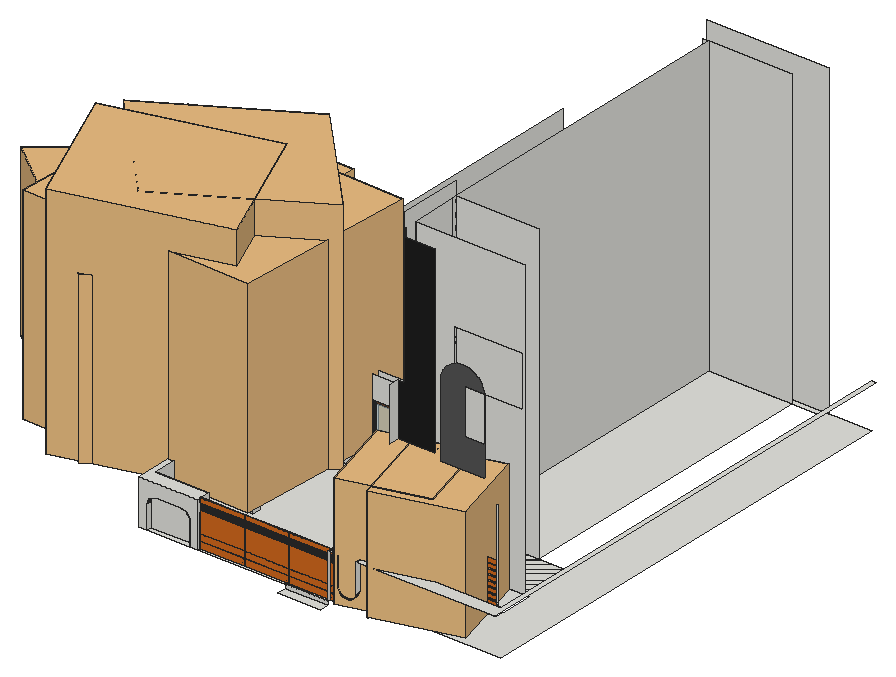
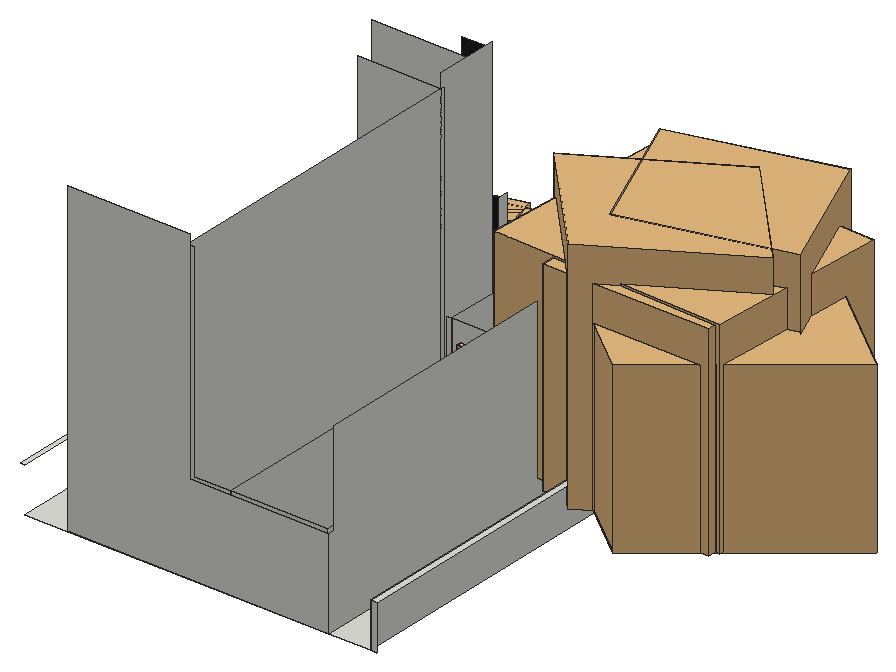
# SketchUp Ruby script. Lengths in inches.
U = 1.inch
M = Sketchup.active_model
def pt(a) = Geom::Point3d.new(a.map { |v| v * U })
def face(e, loops, mat)
  f = e.add_face(loops[0].map { |a| pt(a) })
  loops[1..].each { |l| e.add_face(l.map { |a| pt(a) }).erase! }
  f.material = f.back_material = mat if mat
  f
end
# faces: each face lists its corners as indices into pts; further lists are holes
def faces(e, pts, list, mat = nil) = list.each { |f| face(e, (f[0].is_a?(Array) ? f : [f]).map { |l| l.map { |i| pts[i] } }, mat) }
# xy, xz, yz: faces in a plane at the given z, y or x. An outline is a flat list of corners, or four numbers for a rectangle; further outlines are holes
def ring(l) = l.size == 4 ? [[l[0], l[1]], [l[2], l[1]], [l[2], l[3]], [l[0], l[3]]] : l.each_slice(2).to_a
def flat(e, list, mat, &to3) = list.each { |f| face(e, (f[0].is_a?(Array) ? f : [f]).map { |l| ring(l).map { |u, v| to3.(u, v) } }, mat) }
def xy(e, z, list, mat = nil) = flat(e, list, mat) { |x, y| [x, y, z] }
def xz(e, y, list, mat = nil) = flat(e, list, mat) { |x, z| [x, y, z] }
def yz(e, x, list, mat = nil) = flat(e, list, mat) { |y, z| [x, y, z] }
def lines(e, pts, list) = list.each { |a, b| e.add_line(pt(pts[a]), pt(pts[b])) }
# prism: a flat outline (further loops are holes) pulled along v
def prism(e, loops, v, mat = nil)
  f = face(e, loops, mat); d = Geom::Vector3d.new(v.map { |x| x * U })
  f.pushpull(f.normal.samedirection?(d) ? d.length : -d.length)
end
def box(e, o, s, mat = nil) = prism(e, [[o, [o[0] + s[0], o[1], o[2]], [o[0] + s[0], o[1] + s[1], o[2]], [o[0], o[1] + s[1], o[2]]]], [0, 0, s[2]], mat)
def at(x, y, z, deg = 0) = Geom::Transformation.translation(pt([x, y, z])) * Geom::Transformation.rotation(ORIGIN, Z_AXIS, deg.degrees)
def axes(o, x, y, z) = Geom::Transformation.new([*x, 0, *y, 0, *z, 0, *pt(o).to_a, 1])
def part(name) = M.definitions.add(name)
# library, detail: a bought-in or finely detailed component or shape, given as its bounding box
def library(name, o, s) = part(name).tap { |d| box(d.entities, o, s) }
def detail(e, o, s) = box(e.add_group.entities, o, s)
def put(e, d, t, mat = nil) = e.add_instance(d, t).tap { |i| i.material = mat if mat }
def group(e, t, mat = nil) = e.add_group.tap { |g| g.transformation = t; g.material = mat if mat }.entities
root = M.entities
M.materials.add("[0041_Chocolate]").color = [210, 105, 30]
M.materials.add("[Color M06]").color = [84, 84, 84]
M.materials.add("[Color M08]").color = [30, 30, 30]
M.materials.add("[Translucent Glass Safety]").color = [204, 235, 244]
M.materials["[Translucent Glass Safety]"].alpha = 0.5
M.materials.add("[Wood Veneer 01]").color = [120, 70, 37]
M.materials.add("[Wood Veneer 01]2").color = [94, 55, 29]
c1 = library("Group\#287",[-33.32,-34.9375,32.67],[162.87,159.66,128.34])
c2 = library("Group\#288",[-10.45,-6.67,0],[121.7,116.61,164.95])
c3 = library("Group\#286",[-10.45,-6.67,0],[121.7,116.61,164.95])
c4 = library("Group\#284",[-10.45,-6.67,0],[121.7,116.61,164.95])
c5 = library("Group\#283",[-33.32,-34.9375,32.67],[162.87,159.66,128.34])
c6 = library("Group\#285",[-33.32,-34.9375,81.35],[162.87,159.66,79.66])
c7 = library("Group\#282",[-33.32,-34.9375,77.91],[162.87,159.66,83.1])
c8 = part("Palem Elek")
put(c8.entities,c1,axes([92.2,20.3,-29.73],[0.70711,0.70711,0],[-0.70711,0.70711,0],[0,0,0.91208]))
put(c8.entities,c2,axes([60.27,20.78,0],[1,0,0],[0,1,0],[0,0,0.85762]))
put(c8.entities,c3,at(25.45,60.83,0,-53.5))
put(c8.entities,c4,at(84.4375,135.48,0,-161.4))
put(c8.entities,c5,axes([38.54,105.7,-36.19],[-0.04013,-0.99919,0],[0.99919,-0.04013,0],[0,0,1.11001]))
put(c8.entities,c6,axes([57.15,96.51,-54.45],[-0.02003,-0.49872,0.02965],[0.4996,-0.02007,0],[0.00123,0.03065,0.51628]))
put(c8.entities,c7,axes([74.94,50.39,-54.06],[0.40095,0.29715,0.03075],[-0.29654,0.38966,0.10114],[0.04012,-0.11026,0.54246]))
c9 = part("palem elek\#1")
put(c9.entities,c8,at(-81.14,-74.56,-0.83))
c10 = part("Coqueiro")
put(c10.entities,c9,axes([83.17,89.39,9.5625],[0,1.1016,0],[-1.377,0,0],[0,0,1.39284]))
c11 = part("Slatted screen panel")
xy(c11.entities,0,[[0,0,255.91,1.97]],"[Wood Veneer 01]2")
xy(c11.entities,16.54,[[0,1.18,255.91,1.97]],"[Wood Veneer 01]2")
xy(c11.entities,16.93,[[0,0,255.91,1.18]],"[Wood Veneer 01]2")
xy(c11.entities,17.78,[[0,0,255.91,1.18]],"[Wood Veneer 01]2")
xy(c11.entities,34.45,[[0,0,255.91,1.18]],"[Wood Veneer 01]2")
xy(c11.entities,35.07,[[0,0,255.91,1.18]],"[Wood Veneer 01]2")
xy(c11.entities,89.37,[[0,0,255.91,1.97]],"[Wood Veneer 01]2")
xy(c11.entities,92.91,[[0,0,255.91,1.97]],"[Wood Veneer 01]2")
xy(c11.entities,94.49,[[0,0,255.91,1.97]],"[Wood Veneer 01]2")
xy(c11.entities,97.64,[[0,0,255.91,1.97]],"[Wood Veneer 01]2")
xy(c11.entities,99.21,[[0,0,255.91,1.97]],"[Wood Veneer 01]2")
xy(c11.entities,102.36,[[0,0,255.91,1.97]],"[Wood Veneer 01]2")
xy(c11.entities,103.9375,[[0,0,255.91,1.97]],"[Wood Veneer 01]2")
xy(c11.entities,107.48,[[0,0,255.91,1.97]],"[Wood Veneer 01]2")
xy(c11.entities,119.29,[[0,0,255.91,1.97]],"[Wood Veneer 01]2")
xz(c11.entities,0,[[0,0,255.91,16.93],[0,17.78,255.91,34.45],[0,35.07,255.91,89.37],[0,92.91,255.91,94.49],[0,97.64,255.91,99.21],
  [0,102.36,255.91,103.9375],[0,107.48,255.91,119.29]],"[0041_Chocolate]")
xz(c11.entities,1.18,[[0,16.54,255.91,16.93],[0,16.93,255.91,17.78],[0,34.45,255.91,35.07]],"[Wood Veneer 01]2")
xz(c11.entities,1.97,[[0,0,255.91,1.57],[0,1.57,255.91,5.51],[0,5.51,255.91,7.09],[0,7.09,255.91,11.8125],[0,11.8125,255.91,16.54],
  [0,16.54,255.91,19.69],[0,19.69,255.91,89.37],[0,92.91,255.91,94.49],[0,97.64,255.91,99.21],[0,102.36,255.91,103.9375],
  [0,107.48,255.91,109.84],[0,109.84,255.91,119.29]],"[Wood Veneer 01]2")
yz(c11.entities,0,[[0,0,1.97,1.57],[0,1.57,1.97,5.51],[0,5.51,1.97,7.09],[0,7.09,1.97,11.8125],[0,11.8125,0,16.93,1.18,16.93,1.18,16.54,1.97,16.54,1.97,11.8125],
  [1.18,16.54,1.97,19.69],[0,17.78,0,34.45,1.18,34.45,1.18,35.07,0,35.07,0,89.37,1.97,89.37,1.97,19.69,1.18,19.69,1.18,17.78],[0,92.91,1.97,94.49],[0,97.64,1.97,99.21],[0,102.36,1.97,103.9375],
  [0,107.48,1.97,109.84],[0,109.84,1.97,119.29]],"[Wood Veneer 01]2")
yz(c11.entities,255.91,[[0,0,1.97,1.57],[0,1.57,1.97,5.51],[0,5.51,1.97,7.09],[0,7.09,1.97,11.8125],[0,11.8125,1.97,11.8125,1.97,16.54,1.18,16.54,1.18,16.93,0,16.93],
  [1.18,16.54,1.97,19.69],[0,17.78,1.18,17.78,1.18,19.69,1.97,19.69,1.97,89.37,0,89.37,0,35.07,1.18,35.07,1.18,34.45,0,34.45],[0,92.91,1.97,94.49],[0,97.64,1.97,99.21],[0,102.36,1.97,103.9375],
  [0,107.48,1.97,109.84],[0,109.84,1.97,119.29]],"[Wood Veneer 01]2")
p = [[255.91,1.97,103.9375],[255.91,1.97,107.48],[0,1.97,107.48],[0,1.97,103.9375],[0,1.97,92.91],[0,1.97,89.37],
  [255.91,1.97,99.21],[255.91,1.97,102.36],[255.91,1.97,89.37],[255.91,1.97,92.91],[0,1.97,97.64],[0,1.97,94.49],
  [0,1.97,102.36],[0,1.97,99.21],[255.91,1.97,94.49],[255.91,1.97,97.64],[240.94,0,5.51],[240.94,1.97,5.51]]
lines(c11.entities,p,[[0,1],[2,3],[4,5],[6,7],[8,9],[10,11],[12,13],[14,15],[16,17]])
c12 = part("Group\#3")
g1 = group(c12.entities,at(0,0,0))
xy(g1,0,[[0,0,6,48]],"[Wood Veneer 01]")
xy(g1,4,[[0,4,1.8125,44],[1.8125,4,6,44]])
xy(g1,80,[[0,4,1.8125,44],[1.8125,4,6,44]])
xy(g1,84,[[0,0,6,48]],"[Wood Veneer 01]")
xz(g1,0,[[0,0,6,84]],"[Wood Veneer 01]")
xz(g1,4,[[0,4,1.8125,80],[1.8125,4,6,80]])
xz(g1,44,[[0,4,1.8125,80],[1.8125,4,6,80]])
xz(g1,48,[[0,0,6,84]],"[Wood Veneer 01]")
yz(g1,0,[[[0,0,48,84],[4,4,44,80]]],"[Wood Veneer 01]")
yz(g1,1.8125,[[4,4,44,80]],"[Translucent Glass Safety]")
yz(g1,6,[[[0,0,48,84],[4,4,44,80]]],"[Wood Veneer 01]")
g2 = group(c12.entities,at(0,48,0))
xy(g2,0,[[0,0,6,48]],"[Wood Veneer 01]")
xy(g2,4,[[0,4,1.8125,44],[1.8125,4,6,44]])
xy(g2,80,[[0,4,1.8125,44],[1.8125,4,6,44]])
xy(g2,84,[[0,0,6,48]],"[Wood Veneer 01]")
xz(g2,0,[[0,0,6,84]],"[Wood Veneer 01]")
xz(g2,4,[[0,4,1.8125,80],[1.8125,4,6,80]])
xz(g2,44,[[0,4,1.8125,80],[1.8125,4,6,80]])
xz(g2,48,[[0,0,6,84]],"[Wood Veneer 01]")
yz(g2,0,[[[0,0,48,84],[4,4,44,80]]],"[Wood Veneer 01]")
yz(g2,1.8125,[[4,4,44,80]],"[Translucent Glass Safety]")
yz(g2,6,[[[0,0,48,84],[4,4,44,80]]],"[Wood Veneer 01]")
c13 = library("元件\#5",[-4.39,0,0],[5.37,35.83,90.55])
c14 = library("Palm tree",[-4.09,-4.52,0],[193.52,193.51,258.93])
c15 = part("Palm+Tree")
put(c15.entities,c14,at(25.51,-21.81,0,15))
xy(root,0.73,[[782.4,185.9375,839.42,198.625]])
xy(root,6.125,[[597.05,198.625,653.92,204.875],[664.86,198.625,839.66,217.125],[[593.57,217.125,1056.5,217.125,1056.5,838.14,648.9,838.14,648.9,439.98,767.38,439.98,767.38,397.86,777.42,397.86,777.42,405.05,824.61,405.05,824.61,397.86,844.53,397.86,844.53,406.38,786.21,406.38,786.21,448.51,656.13,448.51,656.13,830.91,992.73,830.91,992.73,336.27,999.52,336.27,999.52,292.45,998.64,292.45,998.64,280.47,897.21,280.47,897.21,292.45,896.71,292.45,896.71,305.58,847.59,305.58,847.59,292.45,836,292.45,836,397.86,824.61,397.86,824.61,405.05,777.42,405.05,777.42,397.86,767.38,397.86,767.38,439.98,648.9,439.98,648.9,838.14,593.57,838.14],[648.9,294.33,661.9,305.58]],[836,292.45,847.59,305.58],[896.71,292.45,897.21,302.46],
  [648.9,294.33,661.9,305.58],[[897.21,302.46,992.73,302.46,992.73,406.38,844.53,406.38,844.53,397.86,836,397.86,836,312.8125,857.24,312.8125,857.24,305.58,897.21,305.58],[844.53,321.34,845.71,397.86]],[897.21,302.46,897.21,305.58,857.24,305.58,857.24,312.8125,845.71,312.8125,845.71,336.27,992.73,336.27,992.73,302.46],[897.21,302.46,897.21,305.58,857.24,305.58,857.24,312.8125,897.21,312.8125,897.21,305.58,992.73,305.58,992.73,302.46],[896.71,302.46,897.21,305.58],
  [836,305.58,847.59,312.8125],[897.21,305.58,897.21,312.8125,845.71,312.8125,845.71,336.27,992.73,336.27,992.73,305.58],[847.59,305.58,857.24,312.8125],[836,312.8125,836,397.86,844.53,397.86,844.53,321.34,845.71,321.34,845.71,312.8125],[844.53,321.34,845.71,397.86],
  [845.71,336.27,992.73,337.5625],[845.71,337.5625,992.73,337.5625,992.73,406.38,844.53,406.38,844.53,399.07,845.71,399.07],[844.53,397.86,845.71,399.07],[786.21,406.38,844.53,830.91],[844.53,406.38,955.73,830.91],
  [656.13,448.51,786.21,830.91]])
xy(root,11.08,[[897.21,280.47,998.64,281.47]],"[0041_Chocolate]")
xy(root,13.1875,[[897.21,280.47,998.64,281.47]],"[0041_Chocolate]")
xy(root,18.14,[[897.21,280.47,998.64,281.47]],"[0041_Chocolate]")
xy(root,20.25,[[897.21,280.47,998.64,281.47]],"[0041_Chocolate]")
xy(root,25.2,[[897.21,280.47,998.64,281.47]],"[0041_Chocolate]")
xy(root,27.3125,[[897.21,280.47,998.64,281.47]],"[0041_Chocolate]")
xy(root,32.27,[[897.21,280.47,998.64,281.47]],"[0041_Chocolate]")
xy(root,34.375,[[897.21,280.47,998.64,281.47]],"[0041_Chocolate]")
xy(root,39.33,[[897.21,280.47,998.64,281.47]],"[0041_Chocolate]")
xy(root,40.13,[[684.87,439.98,732.5,448.51]])
xy(root,41.4375,[[897.21,280.47,998.64,281.47]],"[0041_Chocolate]")
xy(root,46.39,[[897.21,280.47,998.64,281.47]],"[0041_Chocolate]")
xy(root,48,[[607.98,198.625,642.43,204.875]])
xy(root,48.5,[[897.21,280.47,998.64,281.47]],"[0041_Chocolate]")
xy(root,53.45,[[897.21,280.47,998.64,281.47]],"[0041_Chocolate]")
xy(root,55.5625,[[897.21,280.47,998.64,281.47]],"[0041_Chocolate]")
xy(root,60.52,[[897.21,280.47,998.64,281.47]],"[0041_Chocolate]")
xy(root,62.625,[[897.21,280.47,998.64,281.47]],"[0041_Chocolate]")
xy(root,66.125,[[585.4,198.625,664.86,198.625,664.86,217.125,593.57,217.125,593.57,838.14,585.4,838.14],[839.66,198.625,852.79,198.625,852.79,204.875,877.1,204.875,877.1,198.625,1063.02,198.625,1063.02,838.14,1056.5,838.14,1056.5,217.125,839.66,217.125]])
xy(root,74.64,[[897.21,280.47,933.41,281.47]],"[0041_Chocolate]")
xy(root,76.75,[[897.21,280.47,928.32,281.47]],"[0041_Chocolate]")
xy(root,81.7,[[897.21,280.47,921.48,281.47]],"[0041_Chocolate]")
xy(root,83.8125,[[897.21,280.47,919.8,281.47]],"[0041_Chocolate]")
xy(root,88.77,[[897.21,280.47,916.27,281.47]],"[0041_Chocolate]")
xz(root,198.625,[[782.4,0.73,839.42,6.125],[585.4,6.125,597.05,6.125,597.05,37.07,597.14,38.5,597.42,39.9,597.88,41.25,598.51,42.53,599.31,43.72,600.25,44.8,601.32,45.74,602.51,46.54,603.8,47.17,605.15,47.63,606.55,47.91,607.98,48,642.43,48,643.93,47.9,645.4,47.61,646.83,47.125,648.18,46.46,649.43,45.625,650.56,44.63,651.55,43.5,652.38,42.25,653.05,40.9,653.53,39.48,653.82,38.01,653.92,36.51,653.92,6.125,664.86,6.125,664.86,66.125,585.4,66.125]])
xz(root,204.875,[[886.875,0,888.5,55.1875],[597.05,6.125,653.92,6.125,653.92,36.51,653.82,38.01,653.53,39.48,653.05,40.9,652.38,42.25,651.55,43.5,650.56,44.63,649.43,45.625,648.18,46.46,646.83,47.125,645.4,47.61,643.93,47.9,642.43,48,607.98,48,606.55,47.91,605.15,47.63,603.8,47.17,602.51,46.54,601.32,45.74,600.25,44.8,599.31,43.72,598.51,42.53,597.88,41.25,597.42,39.9,597.14,38.5,597.05,37.07]])
xz(root,204.875,[[864.94,16.91,867.74,17.23,870.4,18.17,872.77,19.69,874.74,21.71,876.21,24.11,877.1,26.79,877.1,66.125,852.79,66.125,852.79,26.79,853.67,24.11,855.14,21.71,857.11,19.69,859.49,18.17,862.14,17.23]],"[0041_Chocolate]")
xz(root,217.125,[[593.57,6.125,664.86,66.125]])
xz(root,280.47,[[897.21,13.1875,998.64,18.14],[897.21,20.25,998.64,25.2],[897.21,27.3125,998.64,32.27],[897.21,34.375,998.64,39.33],[897.21,41.4375,998.64,46.39],
  [897.21,48.5,998.64,53.45],[897.21,55.5625,998.64,60.52],[897.21,62.625,998.64,67.58],[897.21,69.6875,998.64,69.6875,998.64,74.64,951.36,74.64,950.09,74.12,942.38,73.1,934.67,74.12,933.41,74.64,897.21,74.64],[897.21,76.75,928.32,76.75,927.49,77.09,921.48,81.7,897.21,81.7],
  [897.21,83.8125,919.8,83.8125,916.59,88,916.27,88.77,897.21,88.77]],"[0041_Chocolate]")
xz(root,281.47,[[897.21,74.64,933.41,74.64,928.32,76.75,897.21,76.75],[897.21,81.7,921.48,81.7,921.32,81.83,919.8,83.8125,897.21,83.8125],[897.21,88.77,916.27,88.77,915.39,90.875,897.21,90.875]],"[0041_Chocolate]")
xz(root,292.45,[[836,6.125,847.59,132.47]])
xz(root,294.33,[[648.9,6.125,661.9,128.75]])
xz(root,295.65,[[[942.38,73.1,950.09,74.12,951.36,74.64,956.45,76.75,957.28,77.09,963.29,81.7,963.45,81.83,964.97,83.8125,968.18,88,968.5,88.77,969.37,90.875,971.16,95.18,971.24,95.83,971.43,97.27,946.98,97.27,946.98,145.27,972.17,145.27,972.17,253.3125,971.52,258.27,971.24,260.375,971.16,261.02,969.37,265.33,968.5,267.4375,968.18,268.21,964.97,272.39,963.45,274.375,963.29,274.5,957.28,279.11,956.45,279.45,951.36,281.5625,950.09,282.09,942.38,283.1,934.67,282.09,933.41,281.5625,928.32,279.45,927.49,279.11,921.48,274.5,921.32,274.375,919.8,272.39,916.59,268.21,916.27,267.4375,915.39,265.33,913.61,261.02,913.53,260.375,913.25,258.27,912.6,253.3125,912.6,102.89,913.25,97.9375,913.53,95.83,913.61,95.18,915.39,90.875,916.27,88.77,916.59,88,919.8,83.8125,921.32,81.83,921.48,81.7,927.49,77.09,928.32,76.75,933.41,74.64,934.67,74.12],[944.83,196.89,971.52,258.27]]],"[Color M06]")
xz(root,302.46,[[896.71,6.125,897.21,8.32],[897.21,6.125,984.18,8.32],[896.71,8.32,897.21,95.62],[897.21,8.32,984.18,126.125]])
xz(root,305.58,[[648.9,6.125,661.9,128.75]])
xz(root,305.58,[[847.59,6.125,896.71,6.125,896.71,126.125,897.21,126.125,897.21,402.64,857.24,402.64,857.24,226.8,847.59,226.8]],"[Color M08]")
xz(root,312.8125,[[845.71,6.125,847.59,126.125],[847.59,6.125,857.24,126.125]])
xz(root,321.34,[[844.53,6.125,845.71,402.64]])
xz(root,337.5625,[[[845.71,6.125,992.73,402.64],[897.21,226.8,990.02,295.72]]])
xz(root,397.86,[[767.38,6.125,777.42,6.125,777.42,101.1875,824.61,101.1875,824.61,6.125,836,6.125,836,126.125,767.38,126.125],[836,6.125,845.71,126.125]])
xz(root,399.07,[[844.53,6.125,845.71,402.64]])
xz(root,405.05,[[777.42,6.125,824.61,101.1875]])
xz(root,406.38,[[844.53,6.125,955.73,402.64]])
xz(root,439.98,[[[648.9,6.125,767.38,126.125],[684.87,40.13,732.5,95.51]]])
xz(root,448.51,[[656.13,6.125,664.65,126.125],[[664.65,6.125,786.21,126.125],[684.87,40.13,732.5,95.51]]])
xz(root,830.91,[[656.13,6.125,786.21,126.125],[786.21,6.125,786.21,126.125,836,126.125,836,402.64,844.53,402.64,844.53,6.125],[844.53,6.125,955.73,402.64]])
xz(root,838.14,[[585.4,6.125,593.57,66.125],[648.9,6.125,648.9,126.125,836,126.125,836,421.25,999.52,421.25,999.52,6.125]])
yz(root,593.57,[[217.125,6.125,838.14,66.125]])
yz(root,597.05,[[198.625,6.125,204.875,37.07]])
yz(root,648.9,[[294.33,6.125,294.33,128.75,298.39,128.75,298.39,126.125,305.58,126.125,305.58,6.125],[439.98,6.125,439.98,252.47,830.91,252.47,830.91,126.125,838.14,126.125,838.14,6.125]])
yz(root,653.92,[[198.625,6.125,204.875,36.51]])
yz(root,656.13,[[448.51,6.125,830.91,126.125]])
yz(root,661.9,[[294.33,6.125,305.58,128.75]])
yz(root,664.86,[[198.625,6.125,217.125,66.125]])
yz(root,684.87,[[439.98,40.13,448.51,95.51]])
yz(root,732.5,[[439.98,40.13,448.51,95.51]])
yz(root,767.38,[[397.86,6.125,439.98,126.125]])
yz(root,777.42,[[397.86,6.125,405.05,101.1875]])
yz(root,786.21,[[406.38,6.125,448.51,126.125],[448.51,6.125,830.91,126.125]])
yz(root,824.61,[[397.86,6.125,405.05,101.1875]])
yz(root,836,[[292.45,6.125,292.45,132.47,305.58,132.47,305.58,126.125,397.86,126.125,397.86,6.125]])
yz(root,839.66,[[198.625,6.125,217.125,66.125]])
yz(root,844.53,[[321.34,6.125,321.34,421.25,406.38,421.25,406.38,402.64,399.07,402.64,399.07,6.125],[399.07,6.125,406.38,402.64],[406.38,6.125,830.91,402.64]])
yz(root,845.71,[[312.8125,6.125,321.34,126.125],[321.34,6.125,336.27,126.125],[336.27,6.125,337.5625,126.125],[337.5625,6.125,397.86,126.125],[397.86,6.125,399.07,6.125,399.07,402.64,337.5625,402.64,337.5625,126.125,397.86,126.125]])
yz(root,847.59,[[292.45,6.125,305.58,226.8]])
yz(root,852.79,[[198.625,26.79,204.875,66.125]])
yz(root,877.1,[[198.625,26.79,204.875,66.125]])
yz(root,888.5,[[203.875,0,204.875,55.1875]])
yz(root,896.71,[[302.46,6.125,305.58,8.32],[302.46,8.32,305.58,95.62]])
yz(root,897.21,[[280.47,6.125,280.47,11.08,281.47,11.08,281.47,13.1875,280.47,13.1875,280.47,18.14,281.47,18.14,281.47,20.25,280.47,20.25,280.47,25.2,281.47,25.2,281.47,27.3125,280.47,27.3125,280.47,32.27,281.47,32.27,281.47,34.375,280.47,34.375,280.47,39.33,281.47,39.33,281.47,41.4375,280.47,41.4375,280.47,46.39,281.47,46.39,281.47,48.5,280.47,48.5,280.47,53.45,281.47,53.45,281.47,55.5625,280.47,55.5625,280.47,60.52,281.47,60.52,281.47,62.625,280.47,62.625,280.47,67.58,281.47,67.58,281.47,69.6875,280.47,69.6875,280.47,74.64,281.47,74.64,281.47,76.75,280.47,76.75,280.47,81.7,281.47,81.7,281.47,83.8125,280.47,83.8125,280.47,88.77,281.47,88.77,281.47,90.875,280.47,90.875,280.47,95.83,281.47,95.83,281.47,97.9375,280.47,97.9375,280.47,102.89,281.47,102.89,281.47,105,280.47,105,280.47,109.95,281.47,109.95,281.47,112.0625,280.47,112.0625,280.47,117.02,281.47,117.02,281.47,119.125,280.47,119.125,280.47,124.08,281.47,124.08,281.47,126.1875,280.47,126.1875,280.47,131.14,281.47,131.14,281.47,133.25,280.47,133.25,280.47,138.2,281.47,138.2,281.47,140.3125,280.47,140.3125,280.47,141.26,292.45,141.26,292.45,126.125,302.46,126.125,302.46,6.125]])
p = [[864.94,204.875,16.91],[862.14,204.875,17.23],[862.14,198.625,17.23],[864.94,198.625,16.91],[867.74,204.875,17.23],[867.74,198.625,17.23],
  [859.49,204.875,18.17],[859.49,198.625,18.17],[870.4,204.875,18.17],[870.4,198.625,18.17],[857.11,204.875,19.69],[857.11,198.625,19.69],
  [872.77,204.875,19.69],[872.77,198.625,19.69],[855.14,204.875,21.71],[855.14,198.625,21.71],[874.74,204.875,21.71],[874.74,198.625,21.71],
  [853.67,204.875,24.11],[853.67,198.625,24.11],[876.21,204.875,24.11],[876.21,198.625,24.11],[852.79,204.875,26.79],[852.79,198.625,26.79],
  [877.1,204.875,26.79],[877.1,198.625,26.79],[653.82,204.875,38.01],[653.92,204.875,36.51],[653.92,198.625,36.51],[653.82,198.625,38.01],
  [597.05,204.875,37.07],[597.14,204.875,38.5],[597.14,198.625,38.5],[597.05,198.625,37.07],[653.53,204.875,39.48],[653.53,198.625,39.48],
  [597.42,204.875,39.9],[597.42,198.625,39.9],[653.05,204.875,40.9],[653.05,198.625,40.9],[597.88,204.875,41.25],[597.88,198.625,41.25],
  [652.38,204.875,42.25],[652.38,198.625,42.25],[598.51,204.875,42.53],[598.51,198.625,42.53],[651.55,204.875,43.5],[651.55,198.625,43.5],
  [599.31,204.875,43.72],[599.31,198.625,43.72],[650.56,204.875,44.63],[650.56,198.625,44.63],[600.25,204.875,44.8],[600.25,198.625,44.8],
  [649.43,204.875,45.625],[649.43,198.625,45.625],[601.32,204.875,45.74],[601.32,198.625,45.74],[648.18,204.875,46.46],[648.18,198.625,46.46],
  [602.51,204.875,46.54],[602.51,198.625,46.54],[603.8,204.875,47.17],[603.8,198.625,47.17],[646.83,204.875,47.125],[646.83,198.625,47.125],
  [645.4,204.875,47.61],[645.4,198.625,47.61],[605.15,204.875,47.63],[605.15,198.625,47.63],[606.55,204.875,47.91],[606.55,198.625,47.91],
  [643.93,204.875,47.9],[643.93,198.625,47.9],[607.98,204.875,48],[607.98,198.625,48],[642.43,204.875,48],[642.43,198.625,48],
  [934.67,295.65,74.12],[934.67,280.47,74.12],[942.38,280.47,73.1],[942.38,295.65,73.1],[950.09,280.47,74.12],[950.09,295.65,74.12],
  [933.41,295.65,74.64],[933.41,281.47,74.64],[933.41,280.47,74.64],[928.32,281.47,76.75],[928.32,295.65,76.75],[927.49,295.65,77.09],
  [927.49,280.47,77.09],[928.32,280.47,76.75],[921.48,295.65,81.7],[921.48,281.47,81.7],[921.48,280.47,81.7],[921.32,281.47,81.83],
  [921.32,295.65,81.83],[919.8,281.47,83.8125],[919.8,295.65,83.8125],[916.59,295.65,88],[916.59,280.47,88],[919.8,280.47,83.8125],
  [916.27,295.65,88.77],[916.27,281.47,88.77],[916.27,280.47,88.77],[915.39,281.47,90.875],[915.39,295.65,90.875],[897.21,312.8125,24.125],
  [897.21,312.8125,6.125],[897.21,321.34,24.125]]
faces(root,p,[[0,1,2,3],[4,0,3,5],[1,6,7,2],[8,4,5,9],[6,10,11,7],[12,8,9,13],[10,14,15,11],[16,12,13,17],
  [14,18,19,15],[20,16,17,21],[18,22,23,19],[24,20,21,25],[26,27,28,29],[30,31,32,33],[34,26,29,35],[31,36,37,32],
  [38,34,35,39],[36,40,41,37],[42,38,39,43],[40,44,45,41],[46,42,43,47],[44,48,49,45],[50,46,47,51],[48,52,53,49],
  [54,50,51,55],[52,56,57,53],[58,54,55,59],[56,60,61,57],[60,62,63,61],[64,58,59,65],[66,64,65,67],[62,68,69,63],
  [68,70,71,69],[72,66,67,73],[70,74,75,71],[76,72,73,77]])
faces(root,p,[[78,79,80,81],[81,80,82,83],[84,85,86,79,78],[87,85,84,88],[89,90,91,87,88],[92,93,94,90,89],[95,93,92,96],[97,95,96,98],
  [99,100,101,97,98],[102,103,104,100,99],[105,103,102,106]],"[Color M06]")
lines(root,p,[[107,108],[107,109]])
put(root,c10,axes([395.82,246.74,29.13],[1.38444,0,0],[0,1.38444,0],[0,0,1.38444]))
put(root,c11,axes([664.96,201.88,6.125],[0.23355,0,0],[0,0.5124,0],[0,0,0.5124]),"[0041_Chocolate]")
put(root,c12,axes([684.87,442.86,40.13],[0,-0.48,0],[0.49609,0,0],[0,0,0.65923]))
put(root,c11,axes([724.73,201.88,6.125],[0.23355,0,0],[0,0.5124,0],[0,0,0.5124]),"[0041_Chocolate]")
put(root,c13,axes([777.42,398.25,6.11],[0,-1.05,0],[1.302,0,0],[0,0,1.05]))
put(root,c11,axes([784.49,201.88,6.125],[0.23355,0,0],[0,0.5124,0],[0,0,0.5124]),"[0041_Chocolate]")
put(root,c15,axes([835.29,212.94,6.125],[0.58344,0,0],[0,0.58344,0],[0,0,0.58344]),"[Color M06]")
put(root,c15,axes([879.11,212.94,6.125],[0.58344,0,0],[0,0.58344,0],[0,0,0.58344]),"[Color M06]")
